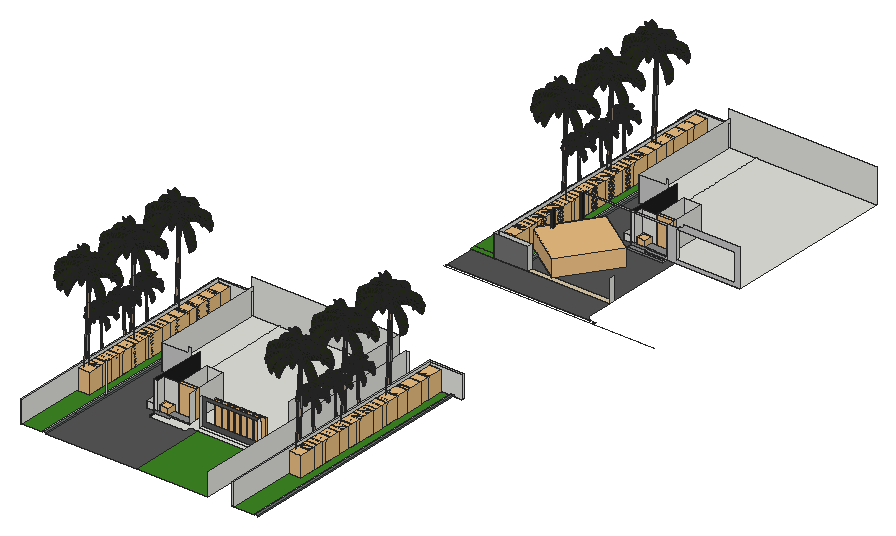
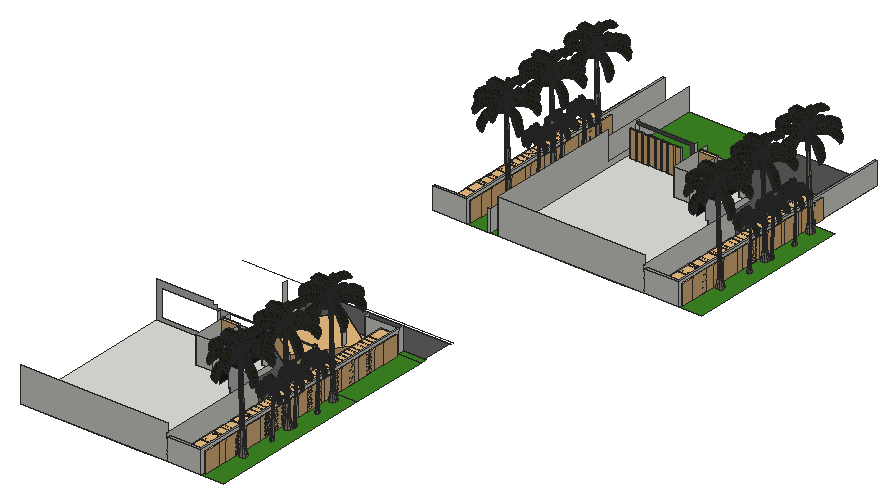
# SketchUp Ruby script. Lengths in inches.
U = 1.inch
M = Sketchup.active_model
def pt(a) = Geom::Point3d.new(a.map { |v| v * U })
def face(e, loops, mat)
  f = e.add_face(loops[0].map { |a| pt(a) })
  loops[1..].each { |l| e.add_face(l.map { |a| pt(a) }).erase! }
  f.material = f.back_material = mat if mat
  f
end
# faces: each face lists its corners as indices into pts; further lists are holes
def faces(e, pts, list, mat = nil) = list.each { |f| face(e, (f[0].is_a?(Array) ? f : [f]).map { |l| l.map { |i| pts[i] } }, mat) }
# xy, xz, yz: faces in a plane at the given z, y or x. An outline is a flat list of corners, or four numbers for a rectangle; further outlines are holes
def ring(l) = l.size == 4 ? [[l[0], l[1]], [l[2], l[1]], [l[2], l[3]], [l[0], l[3]]] : l.each_slice(2).to_a
def flat(e, list, mat, &to3) = list.each { |f| face(e, (f[0].is_a?(Array) ? f : [f]).map { |l| ring(l).map { |u, v| to3.(u, v) } }, mat) }
def xy(e, z, list, mat = nil) = flat(e, list, mat) { |x, y| [x, y, z] }
def xz(e, y, list, mat = nil) = flat(e, list, mat) { |x, z| [x, y, z] }
def yz(e, x, list, mat = nil) = flat(e, list, mat) { |y, z| [x, y, z] }
def lines(e, pts, list) = list.each { |a, b| e.add_line(pt(pts[a]), pt(pts[b])) }
# prism: a flat outline (further loops are holes) pulled along v
def prism(e, loops, v, mat = nil)
  f = face(e, loops, mat); d = Geom::Vector3d.new(v.map { |x| x * U })
  f.pushpull(f.normal.samedirection?(d) ? d.length : -d.length)
end
def box(e, o, s, mat = nil) = prism(e, [[o, [o[0] + s[0], o[1], o[2]], [o[0] + s[0], o[1] + s[1], o[2]], [o[0], o[1] + s[1], o[2]]]], [0, 0, s[2]], mat)
def at(x, y, z, deg = 0) = Geom::Transformation.translation(pt([x, y, z])) * Geom::Transformation.rotation(ORIGIN, Z_AXIS, deg.degrees)
def axes(o, x, y, z) = Geom::Transformation.new([*x, 0, *y, 0, *z, 0, *pt(o).to_a, 1])
def part(name) = M.definitions.add(name)
# library, detail: a bought-in or finely detailed component or shape, given as its bounding box
def library(name, o, s) = part(name).tap { |d| box(d.entities, o, s) }
def detail(e, o, s) = box(e.add_group.entities, o, s)
def put(e, d, t, mat = nil) = e.add_instance(d, t).tap { |i| i.material = mat if mat }
def group(e, t, mat = nil) = e.add_group.tap { |g| g.transformation = t; g.material = mat if mat }.entities
root = M.entities
M.materials.add("Antracyt").color = [44, 47, 50]
M.materials.add("Carpet_Ltblue").color = [157, 173, 165]
M.materials.add("Manila2").color = [36, 43, 22]
M.materials.add("ManilaTruck").color = [158, 143, 128]
M.materials.add("[Color M00]").color = [255, 255, 255]
M.materials.add("[Color M02]").color = [198, 198, 198]
M.materials.add("[Color M04]").color = [60, 133, 34]
M.materials.add("[Color M04]1").color = [142, 142, 142]
M.materials.add("[Color M05]1").color = [114, 114, 114]
M.materials.add("[Color M06]1").color = [86, 86, 86]
M.materials.add("[Color M08]").color = [30, 30, 30]
M.materials.add("[Field Square Tile]").color = [217, 201, 169]
M.materials.add("[Slate Light Tile]").color = [86, 86, 86]
M.materials.add("[Slate]").color = [102, 110, 108]
c1 = part("P_trunck")
xz(c1.entities,2.71,[[7.39,73.15,8.49,73.15,9.26,91.63,8.16,91.63]],"ManilaTruck")
xz(c1.entities,6.09,[[3.91,10.2,7.39,73.15,8.49,73.15,5.33,10.2],[7.39,73.15,8.16,91.63,9.26,91.63,8.49,73.15]],"ManilaTruck")
p = [[3.19,0,0],[3.91,1.7,10.2],[2.75,2.54,10.2],[0.88,1.68,0],[6.05,0,0],[5.33,1.7,10.2],
  [8.36,1.68,0],[6.49,2.54,10.2],[2.31,3.9,10.2],[0,4.39,0],[9.24,4.39,0],[6.93,3.9,10.2],
  [2.75,5.25,10.2],[0.88,7.11,0],[8.36,7.11,0],[6.49,5.25,10.2],[3.91,6.09,10.2],[3.19,8.79,0],
  [6.05,8.79,0],[5.33,6.09,10.2],[7.39,2.71,73.15],[6.5,3.36,73.15],[8.49,2.71,73.15],[9.38,3.36,73.15],
  [6.16,4.4,73.15],[9.72,4.4,73.15],[6.5,5.45,73.15],[9.38,5.45,73.15],[7.39,6.09,73.15],[8.49,6.09,73.15],
  [8.16,2.71,91.63],[7.27,3.36,91.63],[10.15,3.36,91.63],[9.26,2.71,91.63],[6.93,4.4,91.63],[10.49,4.4,91.63],
  [7.27,5.45,91.63],[10.15,5.45,91.63],[8.16,6.09,91.63],[9.26,6.09,91.63]]
faces(c1.entities,p,[[0,1,2,3],[4,5,1,0],[6,7,5,4],[3,2,8,9],[6,10,11,7],[8,12,13,9],[11,10,14,15],[13,12,16,17],
  [18,19,15,14],[17,16,19,18],[1,20,21,2],[5,22,20,1],[7,23,22,5],[2,21,24,8],[7,11,25,23],[8,24,26,12],
  [11,15,27,25],[12,26,28,16],[19,29,27,15],[20,30,31,21],[23,32,33,22],[31,34,24,21],[23,25,35,32],[34,36,26,24],
  [25,27,37,35],[26,36,38,28],[29,39,37,27]],"ManilaTruck")
c2 = part("halfleave")
p = [[3.15,0,0],[0.57,2.5,1.86],[4.875,1.71,0],[46.16,1.62,0],[42.0625,6.98,0],[45.79,16.25,3.85],
  [48.16,12.12,1.98],[48.16,1.62,0],[6.6,3.42,0],[-0.25,5.68,3.48],[9.02,6.6,0],[-0.31,11.68,4.96],
  [2.05,16.625,5.9],[10.99,8.52,0],[36.71,10.67,0],[41.5,21.18,5.01],[8.2,21.17,6.52],[12.96,10.44,0],
  [15.16,24.88,6.8125],[17.61,12.89,0],[31.19,13.02,0],[36.16,23.66,5.26],[19.91,24.88,6.5625],[20.53,13.55,0],
  [25.77,13.9375,0],[30.57,24.88,6.0625],[25.21,24.88,6.26]]
faces(c2.entities,p,[[0,1,2],[3,4,5],[5,6,3],[7,3,6],[2,1,8],[9,8,1],[8,9,10],[11,10,9],
  [11,12,10],[13,10,12],[4,14,15],[15,5,4],[12,16,13],[17,13,16],[16,18,17],[19,17,18],
  [14,20,21],[21,15,14],[18,22,19],[23,19,22],[20,24,25],[25,21,20],[22,26,23],[24,23,26],
  [26,25,24]],"Manila2")
c3 = part("palmfronmanila")
put(c3.entities,c2,axes([0,0,4.06],[1,0,0],[0,1,0],[0,0,-1]))
put(c3.entities,c2,at(0,0,4.06))
c4 = part("manilafronnew")
put(c4.entities,c3,axes([0,16.76,11.56],[1,0,0],[0,0,1],[0,-1,0]))
c5 = part("Palm tree \#1")
put(c5.entities,c1,axes([-10.55,-3.84,0],[1.24992,0,0],[0,1.28016,0],[0,0,1.424]))
g1 = group(c5.entities,at(-43.54,-39.32,114.59))
put(g1,c4,axes([4.6,65.71,26.23],[0.53953,-0.65683,-0.22776],[0.61942,0.58508,-0.22],[0.31564,-0.02543,0.82105]))
put(g1,c4,axes([82.14,44.18,-7.44],[-0.84198,0.16366,0.22983],[-0.16944,-0.87168,0],[0.22561,-0.04385,0.85774]))
put(g1,c4,axes([74.79,11.41,2.76],[-0.448,0.77596,0],[-0.77596,-0.448,0],[0,0,0.896]))
put(g1,c4,axes([70.64,6.04,20.22],[-0.30809,0.82895,-0.08038],[-0.79676,-0.31832,-0.22889],[-0.24248,-0.00729,0.85422]))
put(g1,c4,axes([56.04,79.09,38.5],[-0.31814,-0.55104,-0.36736],[0.63629,-0.36736,0],[-0.18368,-0.31814,0.63629]))
put(g1,c4,axes([8.39,50.1,50.01],[0.44591,-0.25744,-0.51489],[0.36408,0.63061,0],[0.44591,-0.25744,0.51489]))
put(g1,c4,axes([8.53,12.03,22.52],[0.79394,0.3635,-0.23397],[-0.37632,0.82195,0],[0.21274,0.0974,0.8732]))
put(g1,c4,axes([54.07,81.55,-7.16],[-0.44094,-0.76373,0.19874],[0.78289,-0.452,0],[0.09937,0.17211,0.88188]))
put(g1,c4,axes([11.98,71.79,5.35],[0.444,-0.76903,0],[0.76903,0.444,0],[0,0,0.888]))
put(g1,c4,axes([-0.47,46.08,5.17],[0.83758,-0.34011,0],[0.34011,0.83758,0],[0,0,0.904]))
put(g1,c4,axes([35.85,3.71,-10.8],[0.42686,0.73934,0.2973],[-0.78289,0.452,0],[-0.14865,-0.25747,0.85372]))
put(g1,c4,axes([0.28,29.91,5.17],[0.904,0,0],[0,0.904,0],[0,0,0.904]))
put(g1,c4,axes([82.45,61.59,11.57],[-0.88287,-0.17622,-0.08182],[0.17259,-0.88617,0.04625],[-0.08923,0.02954,0.8991]))
put(g1,c4,axes([59.47,9.58,46.3125],[-0.10851,0.51281,-0.52416],[-0.72522,-0.15346,0],[-0.10851,0.51281,0.52416]))
c6 = part("עצי+דקל")
put(c6.entities,c5,axes([111.95,22.91,0],[1.33,0,0],[0,1.33,0],[0,0,1.33]))
put(c6.entities,c5,axes([230.0625,22.91,0],[1.33,0,0],[0,1.33,0],[0,0,1.33]))
put(c6.entities,c5,axes([348.17,22.91,0],[1.33,0,0],[0,1.33,0],[0,0,1.33]))
c7 = library("plant (1)",[-35.72,-28.42,0],[66.31,67.39,84.38])
c8 = library("建立群組\#17",[-3.75,-3.74,-0.43],[25.39,25.39,17.69])
c9 = library("modern+door",[0,0,0],[59.06,11.8125,86.61])
c10 = library("Group\#1",[0,0,0],[29.75,5.78,110.95])
c11 = library("002+Bmw+M4+++mat3.4+2017",[-252.8,19.48,9.01],[196.94,171.32,55.15])
xy(root,-19.75,[[165.7,164.82,173.14,164.82,173.14,1192.15,310.02,1192.15,310.02,1201.875,165.7,1201.875],[1052.17,164.82,1059.6,164.82,1059.6,1192.15,1196.48,1192.15,1196.48,1201.875,1052.17,1201.875],[468.02,464.0625,618.43,464.0625,618.43,487.3125,923.77,487.3125,923.77,1201.875,424.39,1201.875,424.39,505.3125,468.02,505.3125],[310.02,726.125,424.39,1201.875],[684.43,1995.38,691.87,2016.82],
  [691.87,1995.38,827.12,2016.82],[684.43,2016.82,691.87,2016.82,691.87,3044.15,828.75,3044.15,828.75,3053.87,684.43,3053.87],[782.875,2174.7,789.61,2186.43],[986.75,2316.06,1137.16,2316.06,1137.16,2339.31,1442.5,2339.31,1442.5,3053.87,943.125,3053.87,943.125,2357.31,986.75,2357.31],[782.875,2327.31,789.61,2339.31],
  [828.75,2578.12,943.125,3053.87]])
xy(root,-19.75,[[173.14,164.82,260.77,1192.15],[653.09,164.82,951.9375,164.82,951.9375,1201.875,923.77,1201.875,923.77,487.3125,653.09,487.3125],[1059.6,164.82,1147.23,1192.15],[68.91,505.3125,165.7,1201.875],[955.37,505.3125,1052.17,1201.875],
  [587.64,1995.38,684.43,2016.82],[587.64,2016.82,684.43,2357.31],[691.87,2016.82,779.5,3044.15],[587.64,2357.31,684.43,3053.87]],"[Color M04]")
xy(root,-19.75,[[827.12,1995.38,1171.82,2016.82]],"[Field Square Tile]")
xy(root,-19.75,[[274.58,164.82,653.09,164.82,653.09,487.3125,618.43,487.3125,618.43,464.0625,468.02,464.0625,468.02,505.3125,424.39,505.3125,424.39,726.125,310.02,726.125,310.02,1192.15,274.58,1192.15],[594.72,1864.38,1196.62,1864.38,1193.88,1865.28,1189.27,1867.54,1185.03,1870.43,1181.22,1873.89,1177.94,1877.84,1175.25,1882.22,1173.2,1886.93,1171.82,1891.88,1171.82,1995.38,594.72,1995.38],[793.3125,2016.82,1171.82,2016.82,1171.82,2339.31,1137.16,2339.31,1137.16,2316.06,986.75,2316.06,986.75,2357.31,943.125,2357.31,943.125,2578.12,828.75,2578.12,828.75,3044.15,793.3125,3044.15]],"[Slate Light Tile]")
xy(root,-15.625,[[[260.77,164.82,274.58,1192.15],[264.14,475.3125,270.875,487.3125],[264.14,322.71,270.875,334.4375]],[[1147.23,164.82,1161.04,1192.15],[1150.61,475.3125,1157.34,487.3125],[1150.61,322.71,1157.34,334.4375]],[[779.5,2016.82,793.3125,3044.15],[782.875,2327.31,789.61,2339.31],[782.875,2174.7,789.61,2186.43]]],"[Slate]")
xy(root,-14.01,[[986.75,2316.06,1137.16,2316.06,1137.16,2326.56,1052.79,2326.56,1052.79,2339.31,986.75,2339.31]],"[Color M04]1")
xy(root,-8.01,[[1052.79,2326.56,1137.16,2339.31]],"[Color M04]1")
xy(root,-3.75,[[658.22,487.3125,903.98,498.6875]])
xy(root,-2.375,[[483.31,487.3125,618.43,487.3125,618.43,662.5,548.21,662.5,548.21,521.5625,483.31,521.5625],[1002.04,2339.31,1137.16,2339.31,1137.16,2514.49,1066.94,2514.49,1066.94,2373.56,1002.04,2373.56]],"[Color M04]1")
xz(root,487.3125,[[264.14,-15.625,270.875,110.1875],[468.02,-2.375,483.31,110.1875]])
xz(root,487.3125,[[468.02,-14.01,534.06,-14.01,534.06,-8.01,618.43,-8.01,618.43,-2.375,468.02,-2.375]],"[Color M04]1")
xz(root,498.6875,[[658.22,-3.75,903.98,-3.75,903.98,18.41,677.53,18.41,677.53,97.03,903.98,97.03,903.98,110.1875,658.22,110.1875]],"[Color M06]1")
xz(root,505.3125,[[424.39,-19.75,468.02,5.0625]])
xz(root,521.5625,[[483.31,-2.375,548.21,110.1875]])
xz(root,662.5,[[548.21,-2.375,618.43,110.1875]])
xz(root,726.125,[[310.02,-19.75,424.39,-19.75,424.39,5.0625,429.58,5.0625,429.58,110.1875,424.39,110.1875,424.39,88,310.02,88]],"[Color M02]")
xz(root,1192.15,[[173.14,-19.75,260.77,-19.75,260.77,-15.625,274.58,-15.625,274.58,-19.75,310.02,-19.75,310.02,73,173.14,73],[260.77,-19.75,274.58,-15.625],[1059.6,-19.75,1147.23,-19.75,1147.23,-15.625,1161.04,-15.625,1161.04,-19.75,1196.48,-19.75,1196.48,73,1059.6,73],[1147.23,-19.75,1161.04,-15.625]])
xz(root,1201.875,[[165.7,-19.75,310.02,73],[310.02,-19.75,310.02,88,306.21,88,306.21,125.0625,923.77,125.0625,923.77,-19.75],[951.9375,-19.75,962.46,73],[1052.17,-19.75,1196.48,73]])
xz(root,1864.38,[[594.72,-19.75,1219.05,-19.3125]])
xz(root,1995.38,[[684.43,-19.75,827.12,73]],"[Color M05]1")
xz(root,2016.82,[[684.43,-19.75,691.87,73],[691.87,-19.75,691.87,73,827.12,73,827.12,-19.75,793.3125,-19.75,793.3125,-15.625,779.5,-15.625,779.5,-19.75],[779.5,-19.75,793.3125,-15.625]])
xz(root,2174.7,[[782.875,-19.75,789.61,-15.625]])
xz(root,2174.7,[[782.875,-15.625,789.61,115.91]],"[Color M08]")
xz(root,2186.43,[[782.875,-19.75,789.61,-15.625],[782.875,-15.625,789.61,115.91]])
xz(root,2316.06,[[986.75,-19.75,1137.16,-14.01]],"[Color M04]1")
xz(root,2326.56,[[1052.79,-14.01,1137.16,-8.01]],"[Color M04]1")
xz(root,2327.31,[[782.875,-19.75,789.61,-15.625]])
xz(root,2327.31,[[782.875,-15.625,789.61,115.91]],"[Color M08]")
xz(root,2339.31,[[782.875,-19.75,789.61,-15.625],[782.875,-15.625,789.61,110.1875],[986.75,-2.375,1002.04,110.1875]])
xz(root,2339.31,[[[1137.16,-19.75,1442.5,-19.75,1442.5,136.125,1205.57,136.125,1205.57,125.0625,1189.95,125.0625,1189.95,123.92,1189.64,123.92,1189.64,117.06,1189.95,117.06,1189.95,115.91,794.09,115.91,794.09,110.1875,1137.16,110.1875],[1176.95,-3.75,1422.71,110.1875]]],"[Color M02]")
xz(root,2339.31,[[986.75,-14.01,1052.79,-14.01,1052.79,-8.01,1137.16,-8.01,1137.16,-2.375,986.75,-2.375]],"[Color M04]1")
xz(root,2357.31,[[943.125,-19.75,986.75,5.0625]])
xz(root,2373.56,[[1002.04,-2.375,1066.94,110.1875]])
xz(root,2514.49,[[1066.94,-2.375,1137.16,110.1875]])
xz(root,2578.12,[[828.75,-19.75,943.125,-19.75,943.125,5.0625,948.3125,5.0625,948.3125,110.1875,943.125,110.1875,943.125,88,828.75,88]],"[Color M02]")
xz(root,3044.15,[[691.87,-19.75,779.5,-19.75,779.5,-15.625,793.3125,-15.625,793.3125,-19.75,828.75,-19.75,828.75,73,691.87,73],[779.5,-19.75,793.3125,-15.625]])
xz(root,3053.87,[[684.43,-19.75,828.75,73],[828.75,-19.75,828.75,88,824.9375,88,824.9375,125.0625,1442.5,125.0625,1442.5,-19.75]])
yz(root,165.7,[[164.82,-19.75,1201.875,73]])
yz(root,173.14,[[164.82,-19.75,1192.15,73]])
yz(root,260.77,[[164.82,-19.75,1192.15,-15.625]])
yz(root,274.58,[[164.82,-19.75,1192.15,-15.625]],"[Slate]")
yz(root,310.02,[[726.125,-19.75,726.125,88,1201.875,88,1201.875,73,1192.15,73,1192.15,-19.75]])
yz(root,424.39,[[505.3125,-19.75,726.125,5.0625]])
yz(root,468.02,[[464.0625,-19.75,464.0625,-14.01,487.3125,-14.01,487.3125,110.1875,726.125,110.1875,726.125,5.0625,505.3125,5.0625,505.3125,-19.75]],"[Color M08]")
yz(root,483.31,[[487.3125,-2.375,521.5625,110.1875]])
yz(root,548.21,[[521.5625,-2.375,662.5,110.1875]])
yz(root,618.43,[[487.3125,-2.375,662.5,110.1875]])
yz(root,658.22,[[487.3125,-3.75,498.6875,110.1875]])
yz(root,684.43,[[1995.38,-19.75,2016.82,73],[2016.82,-19.75,3053.87,73]])
yz(root,691.87,[[2016.82,-19.75,3044.15,73]])
yz(root,779.5,[[2016.82,-19.75,3044.15,-15.625]])
yz(root,782.875,[[2174.7,-19.75,2186.43,-15.625],[2327.31,-19.75,2339.31,-15.625],[2174.7,-15.625,2186.43,115.66],[2327.31,-15.625,2339.31,115.66]])
yz(root,789.61,[[2174.7,-19.75,2186.43,-15.625],[2327.31,-19.75,2339.31,-15.625]])
yz(root,789.61,[[2174.7,-15.625,2186.43,115.91],[2327.31,-15.625,2339.31,115.91]],"[Color M08]")
yz(root,793.3125,[[2016.82,-19.75,3044.15,-15.625]],"[Slate]")
yz(root,827.12,[[1995.38,-19.75,2016.82,73]])
yz(root,828.75,[[2578.12,-19.75,2578.12,88,3053.87,88,3053.87,73,3044.15,73,3044.15,-19.75]])
yz(root,903.98,[[487.3125,-3.75,487.3125,110.1875,498.6875,110.1875,498.6875,97.03,501.72,97.03,501.72,18.41,498.6875,18.41,498.6875,-3.75]],"[Color M00]")
yz(root,923.77,[[487.3125,-19.75,1201.875,-19.75,1201.875,125.0625,623.84,125.0625,623.84,5.0625,487.3125,5.0625]])
yz(root,943.125,[[2357.31,-19.75,2578.12,5.0625]])
yz(root,951.9375,[[164.82,-19.75,1201.875,73]])
yz(root,986.75,[[2316.06,-19.75,2316.06,-14.01,2339.31,-14.01,2339.31,110.1875,2578.12,110.1875,2578.12,5.0625,2357.31,5.0625,2357.31,-19.75]],"[Color M08]")
yz(root,1002.04,[[2339.31,-2.375,2373.56,110.1875]])
yz(root,1052.17,[[164.82,-19.75,1201.875,73]])
yz(root,1052.79,[[2326.56,-14.01,2339.31,-8.01]])
yz(root,1059.6,[[164.82,-19.75,1192.15,73]])
yz(root,1066.94,[[2373.56,-2.375,2514.49,110.1875]])
yz(root,1137.16,[[2316.06,-19.75,2339.31,-14.01],[2326.56,-14.01,2339.31,-8.01],[2339.31,-2.375,2514.49,110.1875]])
yz(root,1147.23,[[164.82,-19.75,1192.15,-15.625]])
yz(root,1161.04,[[164.82,-19.75,1192.15,-15.625]],"[Slate]")
yz(root,1171.82,[[1995.38,-19.75,2016.82,73]])
yz(root,1176.95,[[2339.31,-3.75,2350.68,110.1875]])
p = [[587.64,1851.99,-19.3125],[594.72,1851.99,-19.3125],[594.72,1864.38,-19.3125],[594.72,1864.38,-19.75],[587.64,1864.38,-19.75],[1474.1,1851.99,-19.3125],
  [587.64,1864.38,-19.3125]]
lines(root,p,[[0,1],[2,1],[3,4],[1,5],[2,6]])
put(root,c6,at(102.61,983.67,-19.75,-90))
put(root,c6,axes([189.49,332.28,-19.75],[0,2,0],[-2,0,0],[0,0,2]))
put(root,c7,at(193.25,482.67,-19.75))
put(root,c7,at(193.25,526.98,-19.75))
put(root,c7,at(193.25,571.3,-19.75))
put(root,c7,at(193.25,615.61,-19.75))
put(root,c7,at(193.25,659.92,-19.75))
put(root,c7,at(193.25,704.23,-19.75))
put(root,c7,at(193.25,748.55,-19.75))
put(root,c7,at(193.25,792.86,-19.75))
put(root,c7,at(193.25,837.17,-19.75))
put(root,c7,at(193.25,881.48,-19.75))
put(root,c7,at(193.25,935.3,-19.75))
put(root,c7,at(193.25,989.11,-19.75))
put(root,c7,at(193.25,1042.92,-19.75))
put(root,c7,at(193.25,1096.73,-19.75))
put(root,c7,at(193.25,1150.55,-19.75))
put(root,c8,axes([497.28,492.33,-1.8],[1.341,0,0],[0,1.341,0],[0,0,1.341]),"Carpet_Ltblue")
put(root,c9,axes([548.21,519.08,-2.375],[1.21,0,0],[0,1.21,0],[0,0,1.32195]),"Antracyt")
put(root,c6,at(621.34,2835.66,-19.75,-90))
put(root,c6,axes([708.22,2184.28,-19.75],[0,2,0],[-2,0,0],[0,0,2]))
put(root,c10,at(690.55,527.41,-13.92),"[Color M04]")
put(root,c7,at(711.98,2068.79,-19.75))
put(root,c7,at(711.98,2113.1,-19.75))
put(root,c7,at(711.98,2157.42,-19.75))
put(root,c7,at(711.98,2201.73,-19.75))
put(root,c7,at(711.98,2246.04,-19.75))
put(root,c7,at(711.98,2290.35,-19.75))
put(root,c7,at(711.98,2334.67,-19.75))
put(root,c7,at(711.98,2378.98,-19.75))
put(root,c7,at(711.98,2423.29,-19.75))
put(root,c7,at(711.98,2467.6,-19.75))
put(root,c7,at(711.98,2511.92,-19.75))
put(root,c7,at(711.98,2556.23,-19.75))
put(root,c7,at(711.98,2600.54,-19.75))
put(root,c7,at(711.98,2644.85,-19.75))
put(root,c7,at(711.98,2689.17,-19.75))
put(root,c7,at(711.98,2733.48,-19.75))
put(root,c7,at(711.98,2787.29,-19.75))
put(root,c7,at(711.98,2841.1,-19.75))
put(root,c7,at(711.98,2894.92,-19.75))
put(root,c7,at(711.98,2948.73,-19.75))
put(root,c7,at(711.98,3002.54,-19.75))
put(root,c10,at(716.95,528.96,-13.92),"[Color M04]")
put(root,c10,at(743.92,528.96,-13.92),"[Color M04]")
put(root,c10,at(769.98,528.96,-13.92),"[Color M04]")
put(root,c10,at(796.04,528.96,-13.92),"[Color M04]")
put(root,c10,at(822.11,528.96,-13.92),"[Color M04]")
put(root,c10,at(848.17,528.96,-13.92),"[Color M04]")
put(root,c10,at(874.23,528.96,-13.92),"[Color M04]")
put(root,c11,axes([1119.92,2267.91,-31.37],[0.71831,1.07151,0],[-1.07151,0.71831,0],[0,0,1.29]))
put(root,c6,at(989.07,983.67,-19.75,-90))
put(root,c6,axes([1075.95,332.28,-19.75],[0,2,0],[-2,0,0],[0,0,2]))
put(root,c8,axes([1016.02,2344.32,-1.8],[1.341,0,0],[0,1.341,0],[0,0,1.341]),"Carpet_Ltblue")
put(root,c7,at(1079.72,482.67,-19.75))
put(root,c7,at(1079.72,526.98,-19.75))
put(root,c7,at(1079.72,571.3,-19.75))
put(root,c7,at(1079.72,615.61,-19.75))
put(root,c7,at(1079.72,659.92,-19.75))
put(root,c7,at(1079.72,704.23,-19.75))
put(root,c7,at(1079.72,748.55,-19.75))
put(root,c7,at(1079.72,792.86,-19.75))
put(root,c7,at(1079.72,837.17,-19.75))
put(root,c7,at(1079.72,881.48,-19.75))
put(root,c7,at(1079.72,935.3,-19.75))
put(root,c7,at(1079.72,989.11,-19.75))
put(root,c7,at(1079.72,1042.92,-19.75))
put(root,c7,at(1079.72,1096.73,-19.75))
put(root,c7,at(1079.72,1150.55,-19.75))
put(root,c9,axes([1066.94,2371.08,-2.375],[1.21,0,0],[0,1.21,0],[0,0,1.32195]),"Antracyt")
